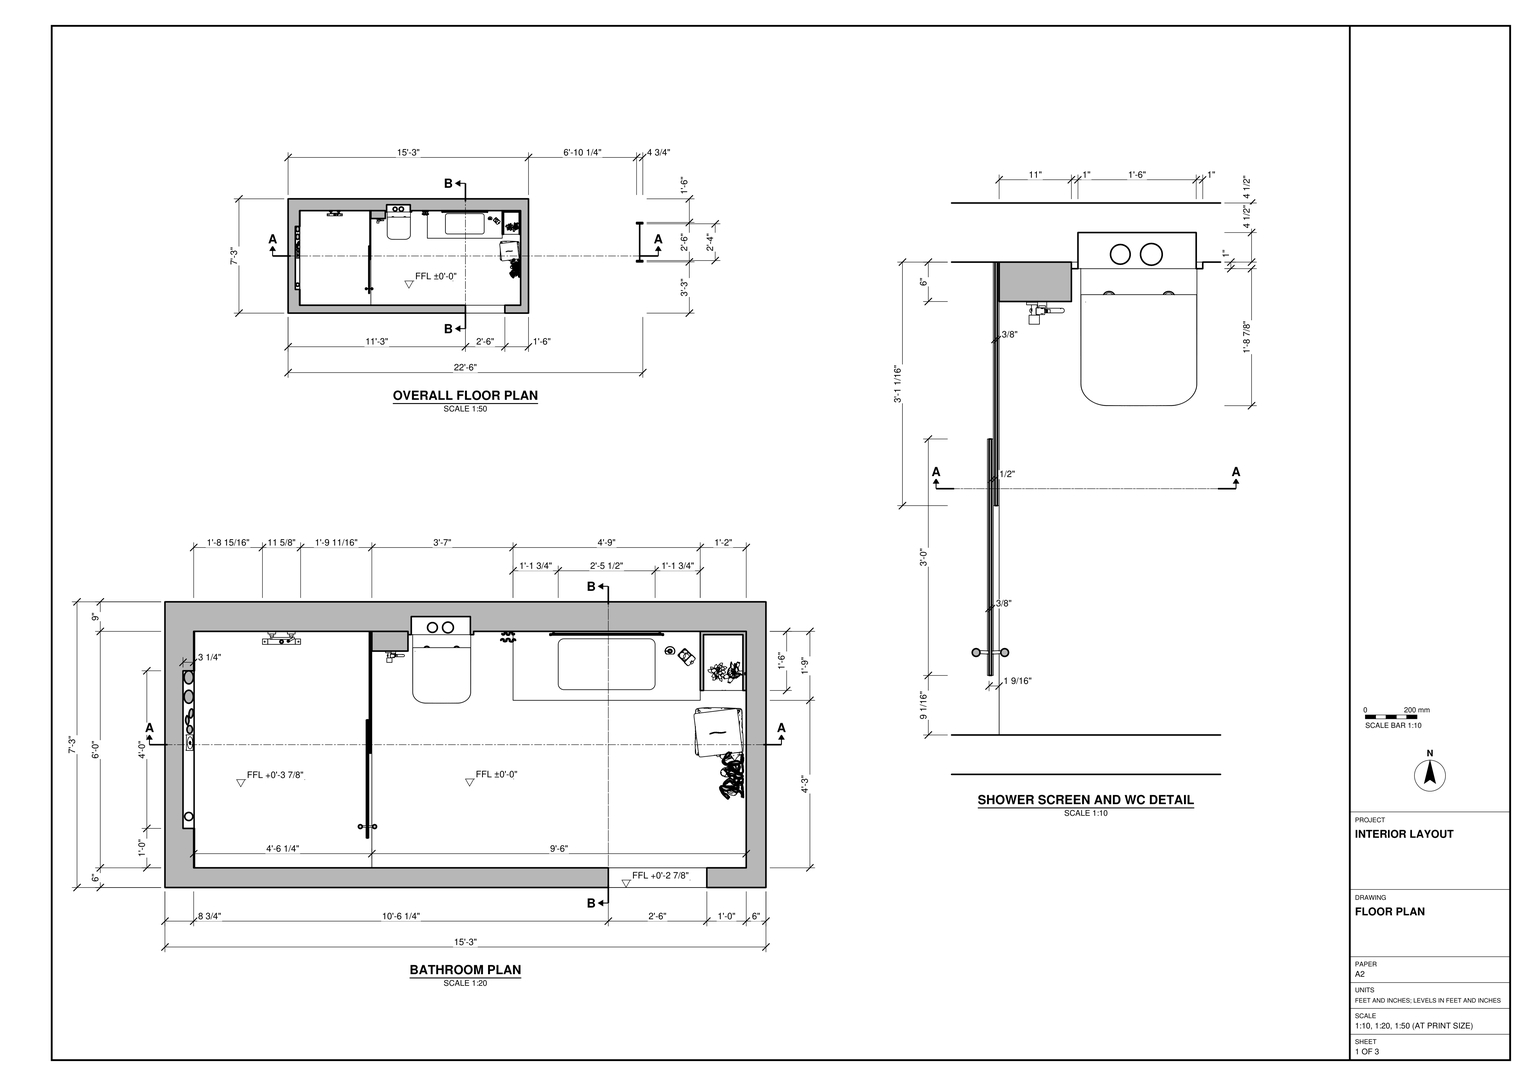
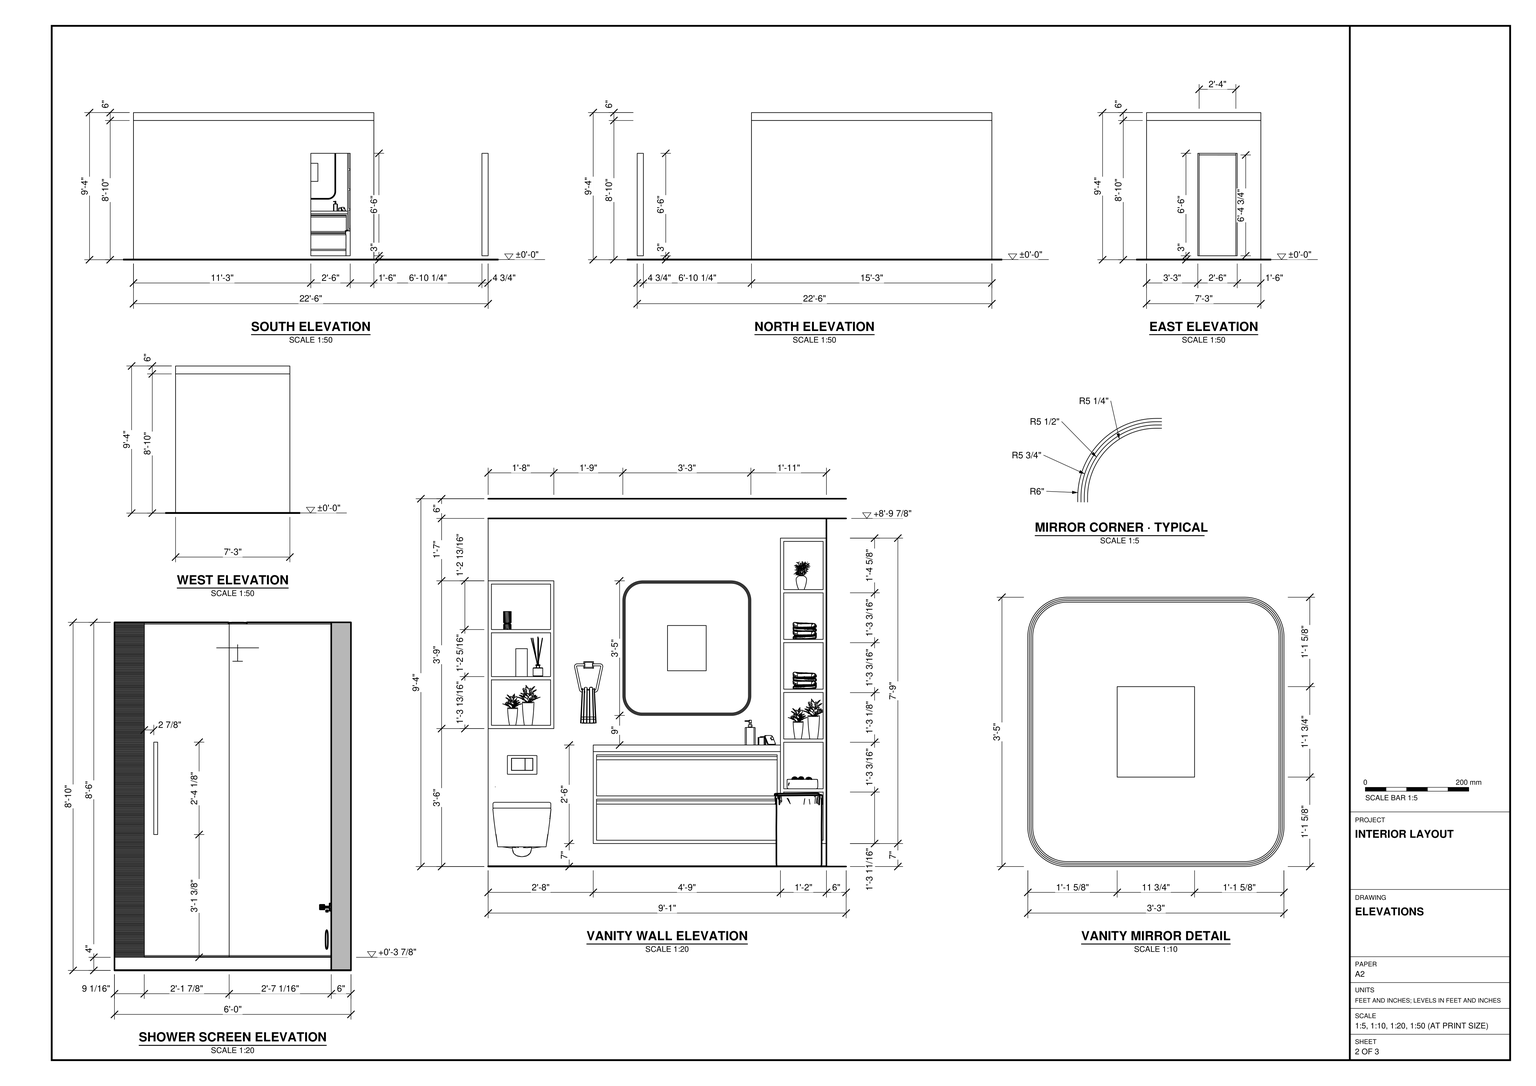
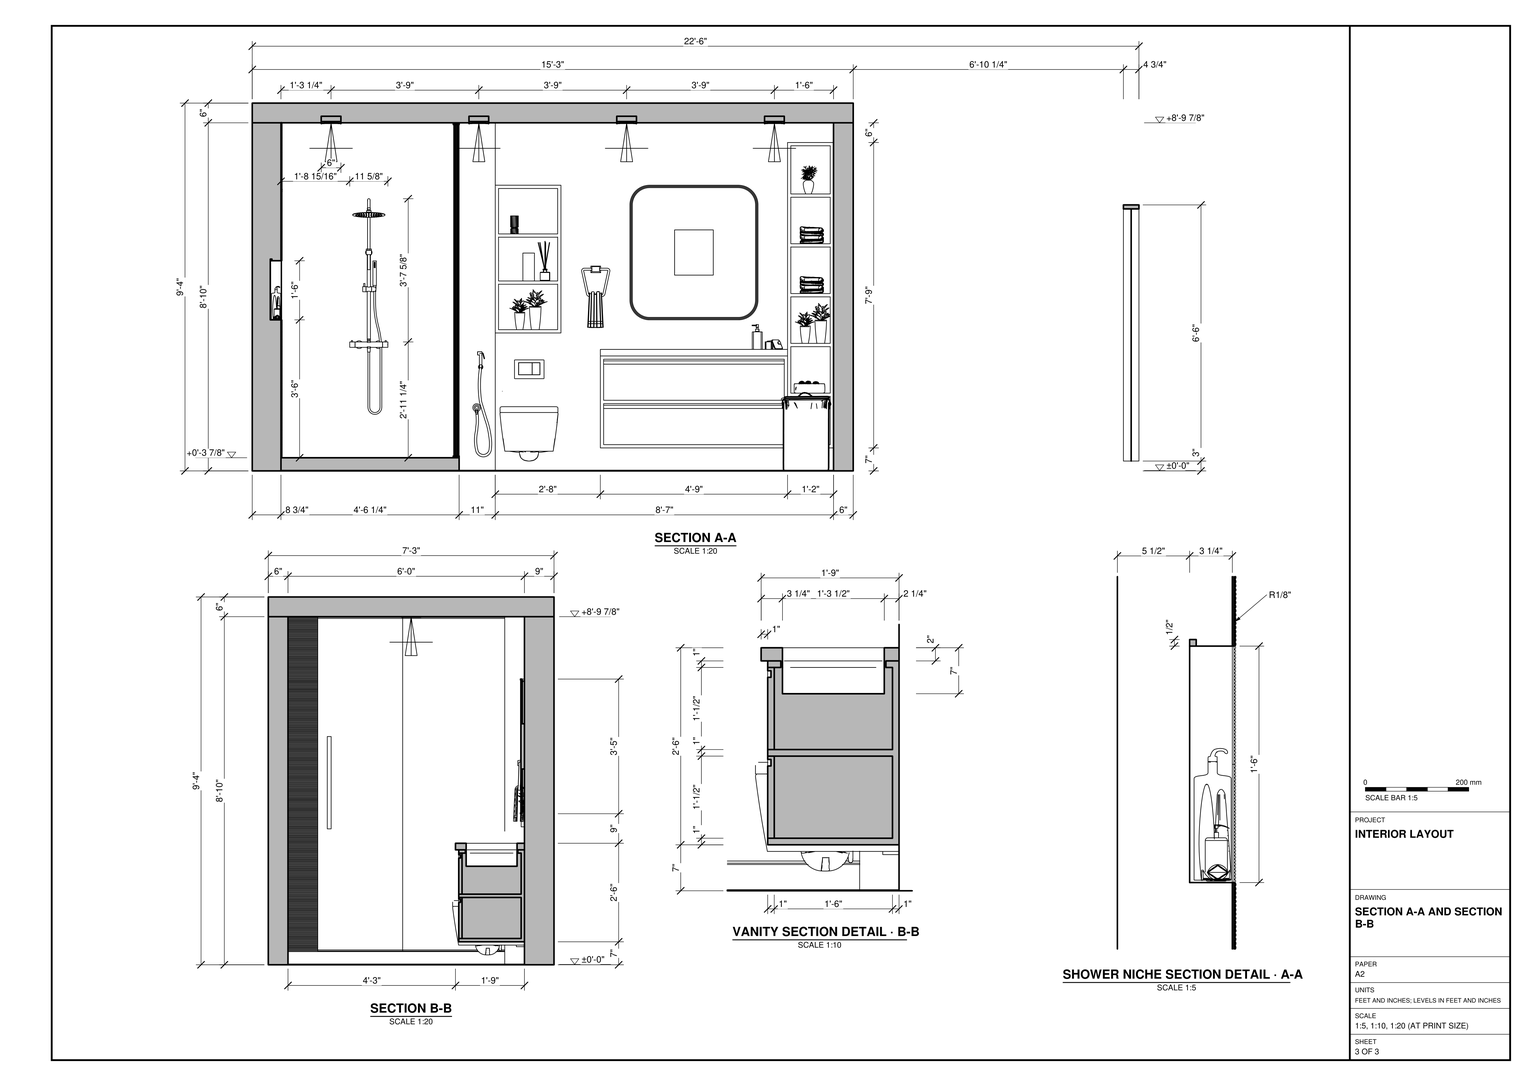
Build the bathroom in SketchUp from task_files/diagram_01.pdf. Work in feet and inches, with the main finished floor at ±0'-0". The complete model is 22'-6" long, 7'-3" deep and 9'-4" high. The bathroom enclosure itself is 15'-3" long; the overall length includes the separate upright panel east of the room. Leave the gap between the enclosure and this panel as drawn.

Use the bathroom plan to set out the perimeter walls at their individual thicknesses, the entrance opening in the south wall and its raised threshold. Model the floor and overhead slab. At the west end, raise the shower floor and enclose it with the glass screen shown in plan and elevation. Include the screen pull, shower fittings and recessed wall niche.

Along the north wall, place the wall-hung toilet beside the screen, with open shelving above it. Model the floating vanity with its inset basin and two drawer fronts, the rounded-corner mirror above it and the tall, narrow shelving unit at the east end. Use the elevations and sections to set their sizes and clearances. Decor and loose items, including towels, baskets, plants and lights, may be any suitable library components placed where shown.

Keep the shell elements and each furniture or joinery piece in separate groups or components, and use components for repeated parts. Save one SketchUp model as output_files/bathroom_interior_with_shower_enclosure_and_vanity_wall.skp.

# SketchUp Ruby script. Lengths in inches.
U = 1.inch
M = Sketchup.active_model
def pt(a) = Geom::Point3d.new(a.map { |v| v * U })
def face(e, loops, mat)
  f = e.add_face(loops[0].map { |a| pt(a) })
  loops[1..].each { |l| e.add_face(l.map { |a| pt(a) }).erase! }
  f.material = f.back_material = mat if mat
  f
end
# faces: each face lists its corners as indices into pts; further lists are holes
def faces(e, pts, list, mat = nil) = list.each { |f| face(e, (f[0].is_a?(Array) ? f : [f]).map { |l| l.map { |i| pts[i] } }, mat) }
# xy, xz, yz: faces in a plane at the given z, y or x. An outline is a flat list of corners, or four numbers for a rectangle; further outlines are holes
def ring(l) = l.size == 4 ? [[l[0], l[1]], [l[2], l[1]], [l[2], l[3]], [l[0], l[3]]] : l.each_slice(2).to_a
def flat(e, list, mat, &to3) = list.each { |f| face(e, (f[0].is_a?(Array) ? f : [f]).map { |l| ring(l).map { |u, v| to3.(u, v) } }, mat) }
def xy(e, z, list, mat = nil) = flat(e, list, mat) { |x, y| [x, y, z] }
def xz(e, y, list, mat = nil) = flat(e, list, mat) { |x, z| [x, y, z] }
def yz(e, x, list, mat = nil) = flat(e, list, mat) { |y, z| [x, y, z] }
def lines(e, pts, list) = list.each { |a, b| e.add_line(pt(pts[a]), pt(pts[b])) }
# prism: a flat outline (further loops are holes) pulled along v
def prism(e, loops, v, mat = nil)
  f = face(e, loops, mat); d = Geom::Vector3d.new(v.map { |x| x * U })
  f.pushpull(f.normal.samedirection?(d) ? d.length : -d.length)
end
def box(e, o, s, mat = nil) = prism(e, [[o, [o[0] + s[0], o[1], o[2]], [o[0] + s[0], o[1] + s[1], o[2]], [o[0], o[1] + s[1], o[2]]]], [0, 0, s[2]], mat)
def at(x, y, z, deg = 0) = Geom::Transformation.translation(pt([x, y, z])) * Geom::Transformation.rotation(ORIGIN, Z_AXIS, deg.degrees)
def axes(o, x, y, z) = Geom::Transformation.new([*x, 0, *y, 0, *z, 0, *pt(o).to_a, 1])
def part(name) = M.definitions.add(name)
# library, detail: a bought-in or finely detailed component or shape, given as its bounding box
def library(name, o, s) = part(name).tap { |d| box(d.entities, o, s) }
def detail(e, o, s) = box(e.add_group.entities, o, s)
def put(e, d, t, mat = nil) = e.add_instance(d, t).tap { |i| i.material = mat if mat }
def group(e, t, mat = nil) = e.add_group.tap { |g| g.transformation = t; g.material = mat if mat }.entities
root = M.entities
M.materials.add("Polis06_194").color = [79, 50, 36]
c1 = library("_CAPIM_DOS_PAMPAS_JULIAAIRES.3D",[-3.51,-2.78,-196.14],[35.86,35.18,43.25])
c2 = library("Group3\#1",[-226.43,63.68,0],[21.09,21.08,29.58])
c3 = library("Plant pots 03",[-13.35,-27.09,0],[26.22,40.73,41.57])
c4 = library("Cesto com toalhas",[0,-0.02,0],[20.47,20.49,27.38])
c5 = part("Bathroom door")
xy(c5.entities,0,[[0,0,4.72,1.18],[0,34.25,4.72,35.43]],"Polis06_194")
xy(c5.entities,85.26,[[0,1.18,4.72,34.25]],"Polis06_194")
xy(c5.entities,86.61,[[0,0,4.72,35.43]],"Polis06_194")
xz(c5.entities,0,[[0,0,4.72,86.61]],"Polis06_194")
xz(c5.entities,1.18,[[0,0,2.36,85.26],[2.36,0,4.72,85.26]],"Polis06_194")
xz(c5.entities,34.25,[[0,0,4.72,85.26]],"Polis06_194")
xz(c5.entities,35.43,[[0,0,4.72,86.61]],"Polis06_194")
yz(c5.entities,0,[[0,0,1.18,86.61],[34.25,0,35.43,86.61],[1.18,85.26,34.25,86.61]],"Polis06_194")
yz(c5.entities,2.36,[[1.18,0,34.25,0,34.25,85.21,1.18,85.26]],"Polis06_194")
yz(c5.entities,4.72,[[0,0,1.18,86.61],[34.25,0,35.43,86.61],[1.18,85.26,34.25,86.61]],"Polis06_194")
c6 = library("Health Faucet",[-0.24,3.23,-9.93],[3.46,9,32.04])
c7 = library("Group\#1",[28.5,-6,0],[183,87,112])
c8 = library("Group\#46",[-1.6,-2.17,0],[14.44,14.68,15.07])
put(root,c1,axes([-191.32,44.09,132.97],[0,-0.31,0],[0.31,0,0],[0,0,0.31]))
put(root,c2,axes([-118.18,-36.89,84.33],[0,-0.3,0],[0.3,0,0],[0,0,0.3]))
put(root,c3,axes([-179.1,40.18,43],[0,-0.3,0],[0.3,0,0],[0,0,0.3]))
put(root,c3,axes([-92.16,26.62,38.83],[0,-0.3,0],[0.3,0,0],[0,0,0.3]))
put(root,c4,axes([-99.83,30.47,8],[0,-0.4625,0],[0.4625,0,0],[0,0,0.4625]))
put(root,c5,axes([0,0,3],[1,0,0],[0,0.84667,0],[0,0,0.90055]))
put(root,c6,at(-201.34,32.76,14.2,-90))
put(root,c7,at(-293.78,-33,0))
put(root,c8,axes([-260.46,-14.75,46],[0,-0.47,0],[0.47,0,0],[0,0,0.47]))
